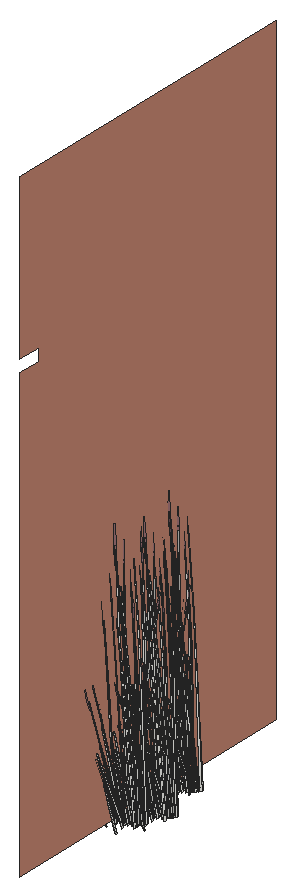
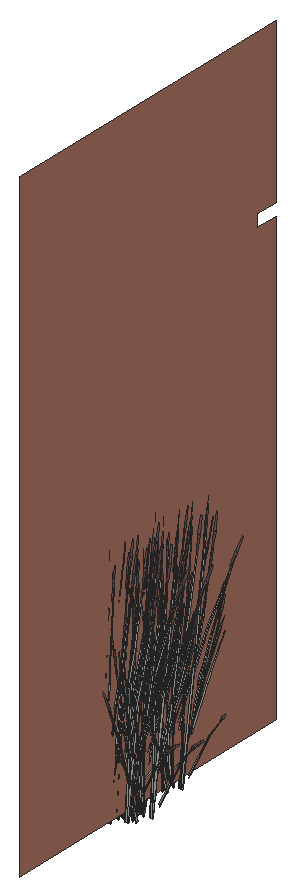
# SketchUp Ruby script. Lengths in inches.
U = 1.inch
M = Sketchup.active_model
def pt(a) = Geom::Point3d.new(a.map { |v| v * U })
def face(e, loops, mat)
  f = e.add_face(loops[0].map { |a| pt(a) })
  loops[1..].each { |l| e.add_face(l.map { |a| pt(a) }).erase! }
  f.material = f.back_material = mat if mat
  f
end
# faces: each face lists its corners as indices into pts; further lists are holes
def faces(e, pts, list, mat = nil) = list.each { |f| face(e, (f[0].is_a?(Array) ? f : [f]).map { |l| l.map { |i| pts[i] } }, mat) }
# xy, xz, yz: faces in a plane at the given z, y or x. An outline is a flat list of corners, or four numbers for a rectangle; further outlines are holes
def ring(l) = l.size == 4 ? [[l[0], l[1]], [l[2], l[1]], [l[2], l[3]], [l[0], l[3]]] : l.each_slice(2).to_a
def flat(e, list, mat, &to3) = list.each { |f| face(e, (f[0].is_a?(Array) ? f : [f]).map { |l| ring(l).map { |u, v| to3.(u, v) } }, mat) }
def xy(e, z, list, mat = nil) = flat(e, list, mat) { |x, y| [x, y, z] }
def xz(e, y, list, mat = nil) = flat(e, list, mat) { |x, z| [x, y, z] }
def yz(e, x, list, mat = nil) = flat(e, list, mat) { |y, z| [x, y, z] }
def lines(e, pts, list) = list.each { |a, b| e.add_line(pt(pts[a]), pt(pts[b])) }
# prism: a flat outline (further loops are holes) pulled along v
def prism(e, loops, v, mat = nil)
  f = face(e, loops, mat); d = Geom::Vector3d.new(v.map { |x| x * U })
  f.pushpull(f.normal.samedirection?(d) ? d.length : -d.length)
end
def box(e, o, s, mat = nil) = prism(e, [[o, [o[0] + s[0], o[1], o[2]], [o[0] + s[0], o[1] + s[1], o[2]], [o[0], o[1] + s[1], o[2]]]], [0, 0, s[2]], mat)
def at(x, y, z, deg = 0) = Geom::Transformation.translation(pt([x, y, z])) * Geom::Transformation.rotation(ORIGIN, Z_AXIS, deg.degrees)
def axes(o, x, y, z) = Geom::Transformation.new([*x, 0, *y, 0, *z, 0, *pt(o).to_a, 1])
def part(name) = M.definitions.add(name)
# library, detail: a bought-in or finely detailed component or shape, given as its bounding box
def library(name, o, s) = part(name).tap { |d| box(d.entities, o, s) }
def detail(e, o, s) = box(e.add_group.entities, o, s)
def put(e, d, t, mat = nil) = e.add_instance(d, t).tap { |i| i.material = mat if mat }
def group(e, t, mat = nil) = e.add_group.tap { |g| g.transformation = t; g.material = mat if mat }.entities
root = M.entities
M.materials.add("Brick_10_1K").color = [200, 136, 115]
M.materials.add("LightPink_Translucent").color = [144, 107, 117]
M.materials["LightPink_Translucent"].alpha = 0.75
c1 = part("blade")
p = [[2.15,0.21,22],[0,0.17,0],[0.09,0.45,0],[2.18,0.31,22],[2.29,0.31,22],[0.38,0.45,0],
  [2.48,0.24,33],[2.49,0.24,33],[2.48,0.22,33]]
faces(c1.entities,p,[[0,1,2,3],[4,5,2,3],[6,3,4,7],[8,0,3,6]])
c2 = part("seeds")
p = [[0.3,-0.1,1.38],[-0.01,-0.03,1.59],[-0.01,-0.03,0.03],[0.14,-0.07,-0.07],[0.29,-0.03,3],[0.15,0.01,3.11]]
faces(c2.entities,p,[[0,1,2,3],[1,0,4,5]],"LightPink_Translucent")
c3 = part("blade with seeds")
put(c3.entities,c1,at(0,0,0))
put(c3.entities,c2,axes([2.4,0.25,30.99],[1.5799,-0.05474,1.17369],[-0.12525,1.92788,0.29478],[-0.07173,-0.02425,1.56792]))
yz(root,342,[[138.72,6,213,6,213,151.99,138.72,151.99,138.72,114,144,114,144,111,138.72,111]],"Brick_10_1K")
put(root,c3,axes([345.02,164.66,6.82],[0.2697,-0.50175,-0.35414],[0.78684,0.14635,0.4572],[-0.07215,-0.20201,0.87481]))
put(root,c3,axes([344.62,165,6.97],[-0.87941,-0.16356,-0.51099],[0.30143,-0.56078,-0.3958],[-0.08064,-0.22578,0.97773]))
put(root,c3,axes([342.87,164.65,7.39],[0.99656,-0.1677,0.53763],[0.17295,0.65785,0.4433],[-0.23438,-0.19388,1.11249]))
put(root,c3,axes([345.37,164.97,7.33],[-0.87543,0.30377,-0.1216],[-0.4302,-0.53915,-0.67495],[-0.1155,-0.2272,1.02557]))
put(root,c3,axes([341.89,164.05,5.06],[0.46666,0.22709,1.1486],[-0.67962,0.13651,0.84392],[-0.14541,-0.17452,0.25299]))
put(root,c3,axes([343.09,164.79,7.02],[0.4066,-0.41448,0.0643],[0.57901,0.24131,0.50621],[-0.18719,-0.13288,0.77189]))
put(root,c3,axes([342.97,167.1,4.39],[-0.36739,-0.66907,-0.69835],[1.05831,-0.24096,-0.18329],[-0.04061,-0.22656,1.54149]))
put(root,c3,axes([345.11,165.18,7.34],[-0.2697,0.50175,0.35414],[-0.78684,-0.14635,-0.4572],[-0.07215,-0.20201,0.87481]))
put(root,c3,axes([344.05,164.39,4.42],[-0.61821,0.37431,-0.03893],[-0.56645,-0.40995,-0.17649],[-0.03988,-0.11616,0.58215]))
put(root,c3,axes([344.84,168.82,5.62],[0.77308,0.2631,1.51261],[-0.75736,0.56681,0.59816],[-0.33924,-0.33594,1.26806]))
put(root,c3,axes([343.22,165.27,7.34],[0.13817,0.52554,0.35414],[-0.78985,0.13877,-0.4572],[-0.21215,-0.1506,0.87481]))
put(root,c3,axes([340.8,167.01,4.3125],[0,-0.65246,-0.49651],[1.00089,0,0],[0,-0.1486,1.57504]))
put(root,c3,axes([341.23,167.02,4.32],[0.62448,-0.40708,-0.30978],[0.62448,0.40708,0.30978],[0,-0.13112,1.38974]))
put(root,c3,axes([343.42,167.76,4.96],[-1.00749,-0.31132,-0.29095],[0.48511,-0.65709,-0.50002],[-0.03166,-0.16133,1.59708]))
put(root,c3,axes([341.42,167.31,4.625],[-0.83213,0.54855,0.30756],[-0.83263,-0.54278,-0.36492],[-0.02906,-0.15578,1.64885]))
put(root,c3,axes([343.67,168.45,4.73],[0.23711,-0.77313,-0.23429],[1.12425,0.13477,0.51271],[-0.19645,-0.10677,1.5644]))
put(root,c3,axes([341.23,167.61,4.77],[0,0.65246,0.49651],[-1.00089,0,0],[0,-0.1486,1.57504]))
put(root,c3,axes([343.59,168.14,4.5],[-0.53742,-0.54764,-0.44739],[0.81403,-0.38564,0.21531],[-0.17391,-0.06776,1.43643]))
put(root,c3,axes([343.51,167.9375,5.01],[-0.43405,0.58792,0.44739],[-0.90188,-0.28295,-0.21531],[0,-0.13553,1.43643]))
put(root,c3,axes([345.38,168.01,4.59],[-0.83213,-0.56158,-0.06131],[0.83263,-0.56193,0],[-0.02906,-0.01961,1.75571]))
put(root,c3,axes([343.8,168.08,4.65],[1.13071,0.13747,0.45755],[-0.23011,0.77639,0.17955],[-0.16524,-0.07497,1.58856]))
put(root,c3,axes([343.19,169.32,4.77],[0.96132,-0.17317,0.17642],[0.23737,0.64447,0.35086],[-0.08574,-0.0939,1.60407]))
put(root,c3,axes([343.98,172.21,4.72],[-0.13683,-0.09148,1.74944],[-0.91315,0.058,-0.27667],[-0.14574,-0.2188,0.14031]))
put(root,c3,axes([344.94,173.76,4.98],[-0.42698,-0.53052,-0.71045],[0.87893,-0.29566,0.08574],[-0.09984,-0.25633,1.00501]))
put(root,c3,axes([344.08,168.63,4.91],[-0.17258,0.58229,0.1448],[-0.84319,-0.10108,-0.41347],[-0.15345,-0.05979,1.26744]))
put(root,c3,axes([346.05,169.35,4.77],[0.25843,-0.64844,0.17642],[0.9457,0.1835,0.35086],[-0.16336,0.00316,1.60407]))
put(root,c3,axes([344.2,172.58,1.49],[-0.15005,0.02351,1.76342],[-0.82981,-0.26461,-0.26939],[0.01392,-0.22072,0.30037]))
put(root,c3,axes([344.43,169.42,4.49],[-0.90188,-0.29293,0],[0.43405,-0.60866,0],[0,0,1.62707]))
put(root,c3,axes([345.18,168.64,4.76],[-0.87356,-0.52515,-0.25192],[0.73507,-0.5897,0.5513],[-0.23523,0.06143,1.68216]))
put(root,c3,axes([342.88,169.65,4.77],[0.83726,0.32623,0.49651],[-0.50045,0.58498,0],[-0.19069,-0.0743,1.57504]))
put(root,c3,axes([345.02,173.31,4.53],[0.2697,-0.50175,-0.35414],[0.78684,0.14635,0.4572],[-0.07215,-0.20201,0.87481]))
put(root,c3,axes([344.62,173.65,4.68],[-0.87941,-0.16356,-0.51099],[0.30143,-0.56078,-0.3958],[-0.08064,-0.22578,0.97773]))
put(root,c3,axes([345.6,168.21,5.01],[0.97146,-0.04028,0.44739],[0.08785,0.66859,-0.21531],[-0.17391,0.06776,1.43643]))
put(root,c3,axes([344.74,168.53,4.5],[-0.97146,0.04028,-0.44739],[-0.08785,-0.66859,0.21531],[-0.17391,0.06776,1.43643]))
put(root,c3,axes([342.87,173.3,5.09],[0.99656,-0.1677,0.53763],[0.17295,0.65785,0.4433],[-0.23438,-0.19388,1.11249]))
put(root,c3,axes([345.37,173.625,5.03],[-0.87543,0.30377,-0.1216],[-0.4302,-0.53915,-0.67495],[-0.1155,-0.2272,1.02557]))
put(root,c3,axes([341.89,172.71,2.77],[0.46666,0.22709,1.1486],[-0.67962,0.13651,0.84392],[-0.14541,-0.17452,0.25299]))
put(root,c3,axes([345.8125,170.08,4.49],[-0.55235,-0.65609,-0.05142],[0.93577,-0.36461,0.51607],[-0.23059,0.06247,1.6363]))
put(root,c3,axes([345.62,168.49,4.91],[0.66093,0.39201,0.1448],[-0.5513,0.44227,-0.41347],[-0.15345,0.05979,1.26744]))
put(root,c3,axes([343.09,173.44,4.73],[0.4066,-0.41448,0.0643],[0.57901,0.24131,0.50621],[-0.18719,-0.13288,0.77189]))
put(root,c3,axes([342.97,175.75,2.1],[-0.36739,-0.66907,-0.69835],[1.05831,-0.24096,-0.18329],[-0.04061,-0.22656,1.54149]))
put(root,c3,axes([346.32,169.7,4.77],[0.83726,-0.32623,0.49651],[0.50045,0.58498,0],[-0.19069,0.0743,1.57504]))
put(root,c3,axes([345.5625,170,4.32],[-0.83462,-0.16144,-0.30978],[0.21015,-0.56852,0.30978],[-0.16826,0.06556,1.38974]))
put(root,c3,axes([345.11,173.84,5.05],[-0.2697,0.50175,0.35414],[-0.78684,-0.14635,-0.4572],[-0.07215,-0.20201,0.87481]))
put(root,c3,axes([345.42,168.35,4.96],[0.10425,0.7445,-0.29095],[-1.08575,0.04502,-0.50002],[-0.19119,0.09917,1.59708]))
put(root,c3,axes([344.05,173.04,2.13],[-0.61821,0.37431,-0.03893],[-0.56645,-0.40995,-0.17649],[-0.03988,-0.11616,0.58215]))
put(root,c3,axes([344.77,168.92,4.35],[-0.60257,0.49041,-0.62353],[-0.74854,-0.44469,-0.16365],[-0.24146,0.12234,1.37633]))
put(root,c3,axes([344.84,177.48,3.33],[0.77308,0.2631,1.51261],[-0.75736,0.56681,0.59816],[-0.33924,-0.33594,1.26806]))
put(root,c3,axes([345.84,169.74,4.625],[1.11998,0.21207,0.30756],[-0.2802,0.75803,-0.36492],[-0.18537,0.09487,1.64885]))
put(root,c3,axes([345.76,170.26,4.3125],[-0.83726,0.32623,-0.49651],[-0.50045,-0.58498,0],[-0.19069,0.0743,1.57504]))
put(root,c3,axes([343.22,173.92,5.05],[0.13817,0.52554,0.35414],[-0.78985,0.13877,-0.4572],[-0.21215,-0.1506,0.87481]))
put(root,c3,axes([340.8,175.66,2.02],[0,-0.65246,-0.49651],[1.00089,0,0],[0,-0.1486,1.57504]))
put(root,c3,axes([341.98,169.46,7.34],[0.60531,-0.34352,0.35414],[0.573,0.39225,-0.4572],[-0.08718,0.19929,0.87481]))
put(root,c3,axes([346.52,170.16,4.67],[0.55932,0.6538,0],[-0.93577,0.36461,-0.51607],[-0.21313,0.08304,1.63711]))
put(root,c3,axes([341.23,175.67,2.03],[0.62448,-0.40708,-0.30978],[0.62448,0.40708,0.30978],[0,-0.13112,1.38974]))
put(root,c3,axes([346.04,167.57,5.13],[-0.02444,-0.61432,1.41272],[1.10603,0.15924,0.59816],[-0.26159,0.33615,1.3335]))
put(root,c3,axes([341.4375,169.77,7.02],[-0.73517,-0.0304,0.0643],[0.02016,-0.45906,0.50621],[-0.07693,0.17585,0.77189]))
put(root,c3,axes([343.42,176.41,2.67],[-1.00749,-0.31132,-0.29095],[0.48511,-0.65709,-0.50002],[-0.03166,-0.16133,1.59708]))
put(root,c3,axes([341.42,175.96,2.33],[-0.83213,0.54855,0.30756],[-0.83263,-0.54278,-0.36492],[-0.02906,-0.15578,1.64885]))
put(root,c3,axes([343.4375,170.48,7.02],[-0.6592,0.22175,0.0643],[-0.32265,-0.40436,0.50621],[0.06366,0.17825,0.77189]))
put(root,c3,axes([341.67,169.95,6.82],[-0.60531,0.34352,-0.35414],[-0.573,-0.39225,0.4572],[-0.08718,0.19929,0.87481]))
put(root,c3,axes([341.6,169.55,7.69],[0.98321,0.03233,-0.13498],[-0.02687,0.61208,-0.74919],[-0.0683,0.23574,1.13838]))
put(root,c3,axes([343.67,170.4375,7.36],[-0.88151,-0.17057,0.53283],[0.30143,-0.56078,0.43934],[0.05297,0.22053,1.10256]))
put(root,c3,axes([343.67,177.11,2.4375],[0.23711,-0.77313,-0.23429],[1.12425,0.13477,0.51271],[-0.19645,-0.10677,1.5644]))
put(root,c3,axes([342.05,171.28,5.06],[-0.02315,-0.38796,1.1486],[0.57853,0.27671,0.84392],[-0.11378,0.18492,0.25299]))
put(root,c3,axes([341.23,176.26,2.48],[0,0.65246,0.49651],[-1.00089,0,0],[0,-0.1486,1.57504]))
put(root,c3,axes([342.27,169.78,7.3],[0.64041,0.4384,-0.5672],[-0.67652,0.38394,-0.43934],[-0.09744,0.22274,1.08528]))
put(root,c3,axes([341.57,170.44,5.12],[0.8127,-0.11554,0.06507],[0.18684,0.46549,-0.86304],[-0.05152,0.23564,0.7736]))
put(root,c3,axes([343.59,176.79,2.21],[-0.53742,-0.54764,-0.44739],[0.81403,-0.38564,0.21531],[-0.17391,-0.06776,1.43643]))
put(root,c3,axes([343.51,176.59,2.72],[-0.43405,0.58792,0.44739],[-0.90188,-0.28295,-0.21531],[0,-0.13553,1.43643]))
put(root,c3,axes([342.07,169.58,7.63],[-0.02328,0.60353,-0.7886],[-0.98022,-0.04053,0.09517],[-0.10344,0.25568,1.11556]))
put(root,c3,axes([339.51,171.17,7],[0.10149,-0.03939,1.77383],[0.83886,0.26202,-0.16761],[-0.01971,0.21816,0.31391]))
put(root,c3,axes([343,169.16,6.17],[-0.0219,-0.25042,1.71376],[0.94901,0.16613,0.13857],[-0.0587,0.35688,0.73262]))
put(root,c3,axes([343.98,179.38,7.01],[-0.13683,-0.09148,1.74944],[-0.91315,0.058,-0.27667],[-0.14574,-0.2188,0.14031]))
put(root,c3,axes([345.38,176.66,2.3],[-0.83213,-0.56158,-0.06131],[0.83263,-0.56193,0],[-0.02906,-0.01961,1.75571]))
put(root,c3,axes([344.94,180.93,7.27],[-0.42698,-0.53052,-0.71045],[0.87893,-0.29566,0.08574],[-0.09984,-0.25633,1.00501]))
put(root,c3,axes([344.2,179.75,3.79],[-0.15005,0.02351,1.76342],[-0.82981,-0.26461,-0.26939],[0.01392,-0.22072,0.30037]))
put(root,c3,axes([343.8,176.73,2.36],[1.13071,0.13747,0.45755],[-0.23011,0.77639,0.17955],[-0.16524,-0.07497,1.58856]))
put(root,c3,axes([345.02,180.48,6.82],[0.2697,-0.50175,-0.35414],[0.78684,0.14635,0.4572],[-0.07215,-0.20201,0.87481]))
put(root,c3,axes([343.19,177.97,2.47],[0.96132,-0.17317,0.17642],[0.23737,0.64447,0.35086],[-0.08574,-0.0939,1.60407]))
put(root,c3,axes([344.62,180.82,6.97],[-0.87941,-0.16356,-0.51099],[0.30143,-0.56078,-0.3958],[-0.08064,-0.22578,0.97773]))
put(root,c3,axes([341.74,170.43,5.66],[0.01966,-0.33682,1.54345],[0.88405,0.17791,0.21329],[-0.0766,0.35897,0.72882]))
put(root,c3,axes([342.87,180.47,7.39],[0.99656,-0.1677,0.53763],[0.17295,0.65785,0.4433],[-0.23438,-0.19388,1.11249]))
put(root,c3,axes([345.37,180.79,7.33],[-0.87543,0.30377,-0.1216],[-0.4302,-0.53915,-0.67495],[-0.1155,-0.2272,1.02557]))
put(root,c3,axes([344.08,177.29,2.62],[-0.17258,0.58229,0.1448],[-0.84319,-0.10108,-0.41347],[-0.15345,-0.05979,1.26744]))
put(root,c3,axes([341.89,179.875,5.06],[0.46666,0.22709,1.1486],[-0.67962,0.13651,0.84392],[-0.14541,-0.17452,0.25299]))
put(root,c3,axes([346.05,178.01,2.47],[0.25843,-0.64844,0.17642],[0.9457,0.1835,0.35086],[-0.16336,0.00316,1.60407]))
put(root,c3,axes([344.43,178.08,2.2],[-0.90188,-0.29293,0],[0.43405,-0.60866,0],[0,0,1.62707]))
put(root,c3,axes([345.18,177.3,2.46],[-0.87356,-0.52515,-0.25192],[0.73507,-0.5897,0.5513],[-0.23523,0.06143,1.68216]))
put(root,c3,axes([342.88,178.3,2.48],[0.83726,0.32623,0.49651],[-0.50045,0.58498,0],[-0.19069,-0.0743,1.57504]))
put(root,c3,axes([343.09,180.61,7.02],[0.4066,-0.41448,0.0643],[0.57901,0.24131,0.50621],[-0.18719,-0.13288,0.77189]))
put(root,c3,axes([342.97,182.92,4.39],[-0.36739,-0.66907,-0.69835],[1.05831,-0.24096,-0.18329],[-0.04061,-0.22656,1.54149]))
put(root,c3,axes([345.11,181.01,7.34],[-0.2697,0.50175,0.35414],[-0.78684,-0.14635,-0.4572],[-0.07215,-0.20201,0.87481]))
put(root,c3,axes([345.6,176.86,2.72],[0.97146,-0.04028,0.44739],[0.08785,0.66859,-0.21531],[-0.17391,0.06776,1.43643]))
put(root,c3,axes([344.74,177.18,2.21],[-0.97146,0.04028,-0.44739],[-0.08785,-0.66859,0.21531],[-0.17391,0.06776,1.43643]))
put(root,c3,axes([344.05,180.21,4.42],[-0.61821,0.37431,-0.03893],[-0.56645,-0.40995,-0.17649],[-0.03988,-0.11616,0.58215]))
put(root,c3,axes([345.8125,178.73,2.19],[-0.55235,-0.65609,-0.05142],[0.93577,-0.36461,0.51607],[-0.23059,0.06247,1.6363]))
put(root,c3,axes([345.62,177.15,2.62],[0.66093,0.39201,0.1448],[-0.5513,0.44227,-0.41347],[-0.15345,0.05979,1.26744]))
put(root,c3,axes([344.84,184.65,5.62],[0.77308,0.2631,1.51261],[-0.75736,0.56681,0.59816],[-0.33924,-0.33594,1.26806]))
put(root,c3,axes([343.22,181.09,7.34],[0.13817,0.52554,0.35414],[-0.78985,0.13877,-0.4572],[-0.21215,-0.1506,0.87481]))
put(root,c3,axes([340.8,182.83,4.3125],[0,-0.65246,-0.49651],[1.00089,0,0],[0,-0.1486,1.57504]))
put(root,c3,axes([346.32,178.36,2.48],[0.83726,-0.32623,0.49651],[0.50045,0.58498,0],[-0.19069,0.0743,1.57504]))
put(root,c3,axes([345.5625,178.65,2.03],[-0.83462,-0.16144,-0.30978],[0.21015,-0.56852,0.30978],[-0.16826,0.06556,1.38974]))
put(root,c3,axes([345.42,177,2.67],[0.10425,0.7445,-0.29095],[-1.08575,0.04502,-0.50002],[-0.19119,0.09917,1.59708]))
put(root,c3,axes([341.23,182.84,4.32],[0.62448,-0.40708,-0.30978],[0.62448,0.40708,0.30978],[0,-0.13112,1.38974]))
put(root,c3,axes([343.42,183.58,4.96],[-1.00749,-0.31132,-0.29095],[0.48511,-0.65709,-0.50002],[-0.03166,-0.16133,1.59708]))
put(root,c3,axes([344.77,177.57,2.06],[-0.60257,0.49041,-0.62353],[-0.74854,-0.44469,-0.16365],[-0.24146,0.12234,1.37633]))
put(root,c3,axes([345.84,178.4,2.33],[1.11998,0.21207,0.30756],[-0.2802,0.75803,-0.36492],[-0.18537,0.09487,1.64885]))
put(root,c3,axes([345.76,178.91,2.02],[-0.83726,0.32623,-0.49651],[-0.50045,-0.58498,0],[-0.19069,0.0743,1.57504]))
put(root,c3,axes([341.42,183.13,4.625],[-0.83213,0.54855,0.30756],[-0.83263,-0.54278,-0.36492],[-0.02906,-0.15578,1.64885]))
put(root,c3,axes([343.67,184.27,4.73],[0.23711,-0.77313,-0.23429],[1.12425,0.13477,0.51271],[-0.19645,-0.10677,1.5644]))
put(root,c3,axes([341.98,178.11,5.05],[0.60531,-0.34352,0.35414],[0.573,0.39225,-0.4572],[-0.08718,0.19929,0.87481]))
put(root,c3,axes([346.52,178.81,2.375],[0.55932,0.6538,0],[-0.93577,0.36461,-0.51607],[-0.21313,0.08304,1.63711]))
put(root,c3,axes([346.04,176.22,2.84],[-0.02444,-0.61432,1.41272],[1.10603,0.15924,0.59816],[-0.26159,0.33615,1.3335]))
put(root,c3,axes([341.4375,178.42,4.73],[-0.73517,-0.0304,0.0643],[0.02016,-0.45906,0.50621],[-0.07693,0.17585,0.77189]))
put(root,c3,axes([341.23,183.43,4.77],[0,0.65246,0.49651],[-1.00089,0,0],[0,-0.1486,1.57504]))
put(root,c3,axes([343.59,183.96,4.5],[-0.53742,-0.54764,-0.44739],[0.81403,-0.38564,0.21531],[-0.17391,-0.06776,1.43643]))
put(root,c3,axes([343.51,183.76,5.01],[-0.43405,0.58792,0.44739],[-0.90188,-0.28295,-0.21531],[0,-0.13553,1.43643]))
put(root,c3,axes([345.38,183.83,4.59],[-0.83213,-0.56158,-0.06131],[0.83263,-0.56193,0],[-0.02906,-0.01961,1.75571]))
put(root,c3,axes([343.4375,179.13,4.73],[-0.6592,0.22175,0.0643],[-0.32265,-0.40436,0.50621],[0.06366,0.17825,0.77189]))
put(root,c3,axes([341.67,178.6,4.53],[-0.60531,0.34352,-0.35414],[-0.573,-0.39225,0.4572],[-0.08718,0.19929,0.87481]))
put(root,c3,axes([341.6,178.21,5.4],[0.98321,0.03233,-0.13498],[-0.02687,0.61208,-0.74919],[-0.0683,0.23574,1.13838]))
put(root,c3,axes([343.67,179.09,5.0625],[-0.88151,-0.17057,0.53283],[0.30143,-0.56078,0.43934],[0.05297,0.22053,1.10256]))
put(root,c3,axes([342.05,179.93,2.77],[-0.02315,-0.38796,1.1486],[0.57853,0.27671,0.84392],[-0.11378,0.18492,0.25299]))
put(root,c3,axes([343.8,183.9,4.65],[1.13071,0.13747,0.45755],[-0.23011,0.77639,0.17955],[-0.16524,-0.07497,1.58856]))
put(root,c3,axes([342.27,178.4375,5],[0.64041,0.4384,-0.5672],[-0.67652,0.38394,-0.43934],[-0.09744,0.22274,1.08528]))
put(root,c3,axes([341.57,179.1,2.82],[0.8127,-0.11554,0.06507],[0.18684,0.46549,-0.86304],[-0.05152,0.23564,0.7736]))
put(root,c3,axes([343.19,185.14,4.77],[0.96132,-0.17317,0.17642],[0.23737,0.64447,0.35086],[-0.08574,-0.0939,1.60407]))
put(root,c3,axes([342.07,178.24,5.34],[-0.02328,0.60353,-0.7886],[-0.98022,-0.04053,0.09517],[-0.10344,0.25568,1.11556]))
put(root,c3,axes([339.51,179.82,4.71],[0.10149,-0.03939,1.77383],[0.83886,0.26202,-0.16761],[-0.01971,0.21816,0.31391]))
put(root,c3,axes([343,177.81,3.875],[-0.0219,-0.25042,1.71376],[0.94901,0.16613,0.13857],[-0.0587,0.35688,0.73262]))
put(root,c3,axes([344.08,184.46,4.91],[-0.17258,0.58229,0.1448],[-0.84319,-0.10108,-0.41347],[-0.15345,-0.05979,1.26744]))
put(root,c3,axes([346.05,185.18,4.77],[0.25843,-0.64844,0.17642],[0.9457,0.1835,0.35086],[-0.16336,0.00316,1.60407]))
put(root,c3,axes([344.43,185.24,4.49],[-0.90188,-0.29293,0],[0.43405,-0.60866,0],[0,0,1.62707]))
put(root,c3,axes([345.18,184.46,4.76],[-0.87356,-0.52515,-0.25192],[0.73507,-0.5897,0.5513],[-0.23523,0.06143,1.68216]))
put(root,c3,axes([342.88,185.47,4.77],[0.83726,0.32623,0.49651],[-0.50045,0.58498,0],[-0.19069,-0.0743,1.57504]))
put(root,c3,axes([341.74,179.09,3.36],[0.01966,-0.33682,1.54345],[0.88405,0.17791,0.21329],[-0.0766,0.35897,0.72882]))
put(root,c3,axes([345.6,184.03,5.01],[0.97146,-0.04028,0.44739],[0.08785,0.66859,-0.21531],[-0.17391,0.06776,1.43643]))
put(root,c3,axes([344.74,184.35,4.5],[-0.97146,0.04028,-0.44739],[-0.08785,-0.66859,0.21531],[-0.17391,0.06776,1.43643]))
put(root,c3,axes([345.8125,185.9,4.49],[-0.55235,-0.65609,-0.05142],[0.93577,-0.36461,0.51607],[-0.23059,0.06247,1.6363]))
put(root,c3,axes([345.62,184.32,4.91],[0.66093,0.39201,0.1448],[-0.5513,0.44227,-0.41347],[-0.15345,0.05979,1.26744]))
put(root,c3,axes([346.32,185.52,4.77],[0.83726,-0.32623,0.49651],[0.50045,0.58498,0],[-0.19069,0.0743,1.57504]))
put(root,c3,axes([345.5625,185.82,4.32],[-0.83462,-0.16144,-0.30978],[0.21015,-0.56852,0.30978],[-0.16826,0.06556,1.38974]))
put(root,c3,axes([345.42,184.17,4.96],[0.10425,0.7445,-0.29095],[-1.08575,0.04502,-0.50002],[-0.19119,0.09917,1.59708]))
